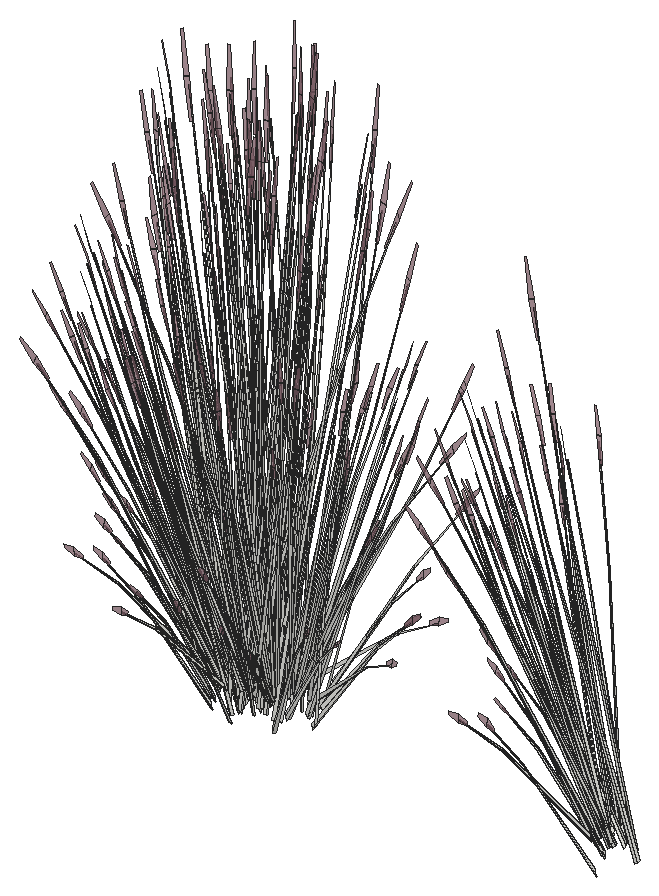
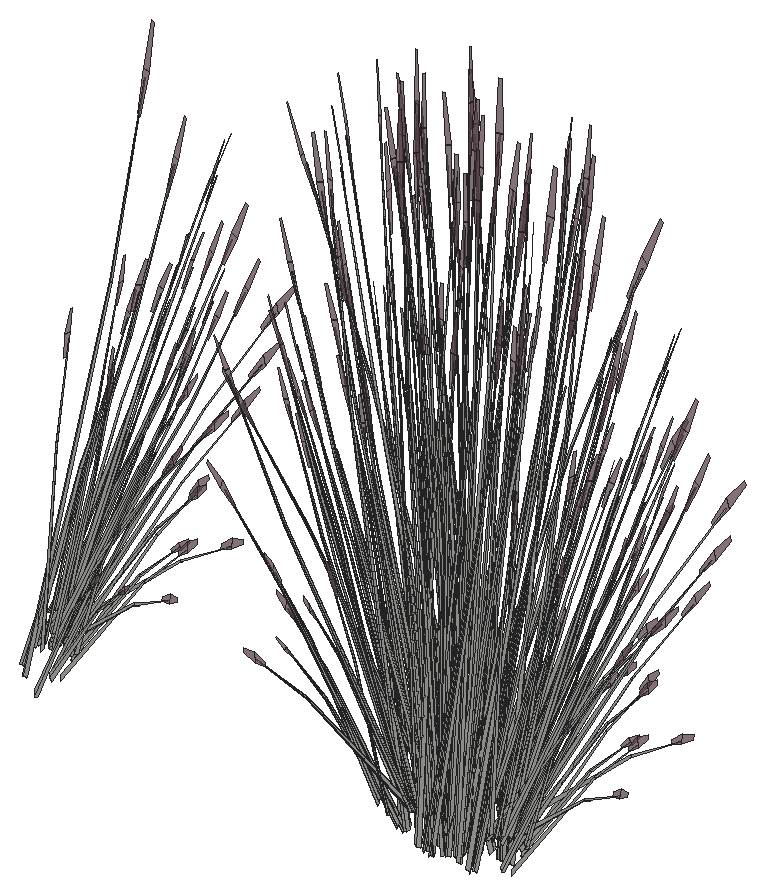
# SketchUp Ruby script. Lengths in inches.
U = 1.inch
M = Sketchup.active_model
def pt(a) = Geom::Point3d.new(a.map { |v| v * U })
def face(e, loops, mat)
  f = e.add_face(loops[0].map { |a| pt(a) })
  loops[1..].each { |l| e.add_face(l.map { |a| pt(a) }).erase! }
  f.material = f.back_material = mat if mat
  f
end
# faces: each face lists its corners as indices into pts; further lists are holes
def faces(e, pts, list, mat = nil) = list.each { |f| face(e, (f[0].is_a?(Array) ? f : [f]).map { |l| l.map { |i| pts[i] } }, mat) }
# xy, xz, yz: faces in a plane at the given z, y or x. An outline is a flat list of corners, or four numbers for a rectangle; further outlines are holes
def ring(l) = l.size == 4 ? [[l[0], l[1]], [l[2], l[1]], [l[2], l[3]], [l[0], l[3]]] : l.each_slice(2).to_a
def flat(e, list, mat, &to3) = list.each { |f| face(e, (f[0].is_a?(Array) ? f : [f]).map { |l| ring(l).map { |u, v| to3.(u, v) } }, mat) }
def xy(e, z, list, mat = nil) = flat(e, list, mat) { |x, y| [x, y, z] }
def xz(e, y, list, mat = nil) = flat(e, list, mat) { |x, z| [x, y, z] }
def yz(e, x, list, mat = nil) = flat(e, list, mat) { |y, z| [x, y, z] }
def lines(e, pts, list) = list.each { |a, b| e.add_line(pt(pts[a]), pt(pts[b])) }
# prism: a flat outline (further loops are holes) pulled along v
def prism(e, loops, v, mat = nil)
  f = face(e, loops, mat); d = Geom::Vector3d.new(v.map { |x| x * U })
  f.pushpull(f.normal.samedirection?(d) ? d.length : -d.length)
end
def box(e, o, s, mat = nil) = prism(e, [[o, [o[0] + s[0], o[1], o[2]], [o[0] + s[0], o[1] + s[1], o[2]], [o[0], o[1] + s[1], o[2]]]], [0, 0, s[2]], mat)
def at(x, y, z, deg = 0) = Geom::Transformation.translation(pt([x, y, z])) * Geom::Transformation.rotation(ORIGIN, Z_AXIS, deg.degrees)
def axes(o, x, y, z) = Geom::Transformation.new([*x, 0, *y, 0, *z, 0, *pt(o).to_a, 1])
def part(name) = M.definitions.add(name)
# library, detail: a bought-in or finely detailed component or shape, given as its bounding box
def library(name, o, s) = part(name).tap { |d| box(d.entities, o, s) }
def detail(e, o, s) = box(e.add_group.entities, o, s)
def put(e, d, t, mat = nil) = e.add_instance(d, t).tap { |i| i.material = mat if mat }
def group(e, t, mat = nil) = e.add_group.tap { |g| g.transformation = t; g.material = mat if mat }.entities
root = M.entities
M.materials.add("LightPink_Translucent").color = [144, 107, 117]
M.materials["LightPink_Translucent"].alpha = 0.75
c1 = part("blade")
p = [[2.15,0.21,22],[0,0.17,0],[0.09,0.45,0],[2.18,0.31,22],[2.29,0.31,22],[0.38,0.45,0],
  [2.48,0.24,33],[2.49,0.24,33],[2.48,0.22,33]]
faces(c1.entities,p,[[0,1,2,3],[4,5,2,3],[6,3,4,7],[8,0,3,6]])
c2 = part("seeds")
p = [[0.3,-0.1,1.38],[-0.01,-0.03,1.59],[-0.01,-0.03,0.03],[0.14,-0.07,-0.07],[0.29,-0.03,3],[0.15,0.01,3.11]]
faces(c2.entities,p,[[0,1,2,3],[1,0,4,5]],"LightPink_Translucent")
c3 = part("blade with seeds")
put(c3.entities,c1,at(0,0,0))
put(c3.entities,c2,axes([2.4,0.25,30.99],[1.5799,-0.05474,1.17369],[-0.12525,1.92788,0.29478],[-0.07173,-0.02425,1.56792]))
put(root,c3,axes([776.41,275.93,1.9375],[0.19062,-0.00741,0.85688],[-0.12645,0.32094,0.06928],[-0.27165,-0.01985,0.36631]))
put(root,c3,axes([776.49,276.49,1.9375],[0.15946,-0.06916,0.85688],[0.13424,0.31957,0.06928],[-0.25033,0.07223,0.36631]))
put(root,c3,axes([776,277.04,1.3],[0.15971,0.02684,0.71501],[0.10294,0.27415,-0.15377],[-0.21694,0.05132,0.3057]))
put(root,c3,axes([777.41,276.16,1.67],[0.13063,-0.0473,0.88532],[0.04505,0.33024,0.06928],[-0.28294,0.04382,0.31642]))
put(root,c3,axes([776,276.38,2.36],[-0.07505,0.04245,0.87472],[0.00638,0.31015,-0.13834],[-0.17202,0.04033,0.07015]))
put(root,c3,axes([776.98,275.63,2.49],[-0.45939,-0.00787,-0.35523],[0.03085,-0.3315,0.04287],[-0.19462,-0.03498,0.5025]))
put(root,c3,axes([776.61,275.71,1.3],[0.08973,0.09103,0.71501],[-0.20675,0.24743,-0.15377],[-0.2123,-0.05914,0.3057]))
put(root,c3,axes([776.25,276.21,2.26],[-0.38192,-0.09121,-0.17707],[0.11139,-0.2661,0.2286],[-0.15377,0.0244,0.4374]))
put(root,c3,axes([776.77,275.42,1.9375],[0.1707,0.05633,0.85688],[-0.35326,0.23632,0.06928],[-0.22018,-0.10661,0.36631]))
put(root,c3,axes([775.17,276.7,2.35],[0.05865,0.00877,0.88692],[0.18143,0.28888,-0.08381],[-0.12006,0.07582,0.15695]))
put(root,c3,axes([776.51,276.34,2.34],[-0.1245,0.29741,-0.25549],[-0.42685,-0.10194,-0.1979],[-0.17186,0.02727,0.48886]))
put(root,c3,axes([776.83,275.7,2.34],[-0.3337,0.21658,-0.25549],[-0.29224,-0.22879,-0.1979],[-0.16955,-0.03295,0.48886]))
put(root,c3,axes([776.29,276.32,0.75],[0.01165,0.05153,0.88171],[-0.23495,0.26909,-0.1347],[-0.16689,-0.01356,0.15018]))
put(root,c3,axes([776.36,275.09,2.35],[0.03407,0.03263,0.88692],[-0.16424,0.29331,-0.08381],[-0.16634,0.00212,0.15695]))
put(root,c3,axes([776.74,274.9,2.36],[-0.09888,-0.00231,0.87472],[-0.3148,0.23079,-0.13834],[-0.16797,-0.04716,0.07015]))
put(root,c3,axes([776.33,276.17,2.37],[0.12984,-0.29812,0.24001],[0.42685,0.10194,0.1979],[-0.16786,0.01792,0.49665]))
put(root,c3,axes([776.49,276.09,2.52],[0.23123,0.29606,-0.0608],[-0.41039,0.14549,-0.33747],[-0.17294,0.03906,0.51278]))
put(root,c3,axes([777.01,275.47,2.52],[-0.02461,0.33251,-0.0608],[-0.4659,-0.00909,-0.33747],[-0.17944,-0.0231,0.51278]))
put(root,c3,axes([776.71,275.5,2.26],[-0.26148,-0.20471,-0.17707],[0.29857,-0.19378,0.2286],[-0.1517,-0.02948,0.4374]))
put(root,c3,axes([776.3,276.09,2.37],[-0.16879,-0.22293,0.03215],[0.30779,-0.10912,0.2531],[-0.13568,0.02153,0.38595]))
put(root,c3,axes([776.08,275.99,1.38],[0.2934,-0.0234,0.5743],[-0.18611,0.20614,0.42196],[-0.14499,-0.03092,0.12649]))
put(root,c3,axes([776.4375,276.92,2.37],[-0.11397,-0.30091,0.24001],[0.44709,-0.05222,0.1979],[-0.13177,0.07077,0.49665]))
put(root,c3,axes([776.67,275.42,2.55],[0.37952,-0.24129,0.26881],[0.32731,0.25625,0.22165],[-0.17806,-0.04451,0.55625]))
put(root,c3,axes([776.35,276.86,2.37],[-0.31549,-0.13751,0.03215],[0.18368,-0.19581,0.2531],[-0.10115,0.06331,0.38595]))
put(root,c3,axes([776.65,276.18,2.53],[0.38192,0.09121,0.17707],[-0.11139,0.2661,-0.2286],[-0.15377,0.0244,0.4374]))
put(root,c3,axes([776.84,275.42,2.37],[0.02314,-0.24862,0.03215],[0.34943,0.00682,0.2531],[-0.13385,-0.02602,0.38595]))
put(root,c3,axes([777.83,276.79,1.03],[-0.47805,-0.0536,-0.31177],[0.10088,-0.33065,-0.08182],[-0.14266,-0.04007,0.68817]))
put(root,c3,axes([777.92,274.99,2.72],[-0.30671,0.31344,-0.0681],[-0.44417,-0.18058,-0.37797],[-0.1544,-0.08856,0.57432]))
put(root,c3,axes([777.08,275.6,2.53],[0.26148,0.20471,0.17707],[-0.29857,0.19378,-0.2286],[-0.1517,-0.02948,0.4374]))
put(root,c3,axes([777.78,275.24,2.49],[-0.39186,-0.15803,-0.35523],[0.27849,-0.27693,0.04287],[-0.14198,-0.09436,0.5025]))
put(root,c3,axes([777.6,275.25,2.34],[-0.45348,0.07772,-0.25549],[-0.07933,-0.29434,-0.1979],[-0.1218,-0.08435,0.48886]))
put(root,c3,axes([777.2,277.42,1.01],[-0.4301,-0.16348,-0.24825],[0.25708,-0.29314,0],[-0.09796,-0.03723,0.78752]))
put(root,c3,axes([777.01,274.98,0.75],[-0.04451,0.04307,0.88171],[-0.44986,0.09286,-0.1347],[-0.10868,-0.08448,0.15018]))
put(root,c3,axes([777.46,277.61,1.1875],[-0.28732,0.32763,0],[-0.4807,-0.18271,-0.25804],[-0.10948,-0.04161,0.81856]))
put(root,c3,axes([776.71,276.82,2.53],[0.40003,-0.04673,0.17707],[0.10563,0.26712,-0.2286],[-0.11464,0.07175,0.4374]))
put(root,c3,axes([776.73,275.15,1.0625],[-0.13257,0.26698,-0.01946],[-0.40802,-0.08212,-0.08825],[-0.06195,-0.04367,0.29107]))
put(root,c3,axes([777.8,274.24,2.35],[-0.00857,0.03919,0.88692],[-0.42284,0.14223,-0.08381],[-0.12443,-0.0727,0.15695]))
put(root,c3,axes([777.34,274.81,1.3],[-0.02783,0.10696,0.71501],[-0.40683,0.08954,-0.15377],[-0.0951,-0.13825,0.3057]))
put(root,c3,axes([777.48,275.09,1.9375],[0.10505,0.10498,0.85688],[-0.48542,0.08838,0.06928],[-0.10971,-0.1648,0.36631]))
put(root,c3,axes([778.37,276.84,1.33],[-0.46399,0.21707,-0.14548],[-0.30855,-0.30672,-0.25001],[-0.11448,-0.03115,0.79854]))
put(root,c3,axes([777.65,275.03,2.26],[-0.07098,-0.26335,-0.17707],[0.40574,-0.06954,0.2286],[-0.10898,-0.07547,0.4374]))
put(root,c3,axes([776.51,276.37,1.1875],[-0.57465,0,0],[0,-0.36542,-0.25804],[0,-0.08323,0.81856]))
put(root,c3,axes([777.32,277.29,1.01],[-0.10795,-0.28489,-0.15489],[0.42874,-0.0809,0.15489],[-0.08643,-0.03285,0.69487]))
put(root,c3,axes([777.89,275.25,2.53],[0.07098,0.26335,0.17707],[-0.40574,0.06954,-0.2286],[-0.10898,-0.07547,0.4374]))
put(root,c3,axes([776.96,276.27,1.17],[-0.42746,0.27488,0.15378],[-0.42772,-0.27199,-0.18246],[-0.01493,-0.07806,0.82443]))
put(root,c3,axes([778.72,277.03,1.66],[0.39713,0.13184,0.7563],[-0.38905,0.28403,0.29908],[-0.17427,-0.16834,0.63403]))
put(root,c3,axes([777.2,274.64,1.38],[0.23972,0.1138,0.5743],[-0.34912,0.06841,0.42196],[-0.0747,-0.08746,0.12649]))
put(root,c3,axes([778.89,276.9375,1.23],[-0.44875,-0.26316,-0.12596],[0.3776,-0.2955,0.27565],[-0.12084,0.03078,0.84108]))
put(root,c3,axes([778.08,276.68,1.11],[-0.27607,-0.27443,-0.2237],[0.41817,-0.19325,0.10766],[-0.08934,-0.03396,0.71822]))
put(root,c3,axes([777.7,274.9375,2.55],[0.51193,-0.08404,0.26881],[0.08885,0.32966,0.22165],[-0.1204,-0.09716,0.55625]))
put(root,c3,axes([778.67,276.88,1.11],[-0.49904,0.02018,-0.2237],[-0.04513,-0.33504,0.10766],[-0.08934,0.03396,0.71822]))
put(root,c3,axes([777.82,275.01,2.37],[0.20887,-0.2077,0.03215],[0.29744,0.12092,0.2531],[-0.09616,-0.06659,0.38595]))
put(root,c3,axes([777.71,277.44,1.24],[0.4301,0.16348,0.24825],[-0.25708,0.29314,0],[-0.09796,-0.03723,0.78752]))
put(root,c3,axes([778.12,276.84,1.22],[0.1218,-0.38743,-0.11714],[0.57753,0.06753,0.25635],[-0.10091,-0.0535,0.7822]))
put(root,c3,axes([778.33,276.93,1.31],[-0.08866,0.29179,0.0724],[-0.43315,-0.05065,-0.20674],[-0.07883,-0.02996,0.63372]))
put(root,c3,axes([778.28,274.39,2.36],[-0.07029,-0.04584,0.87472],[-0.46908,0.02906,-0.13834],[-0.07486,-0.10965,0.07015]))
put(root,c3,axes([776.64,276.12,1.01],[0,-0.32696,-0.24825],[0.51416,0,0],[0,-0.07447,0.78752]))
put(root,c3,axes([776.86,276.42,1.24],[0,0.32696,0.24825],[-0.51416,0,0],[0,-0.07447,0.78752]))
put(root,c3,axes([779.22,277.66,1.1],[-0.28374,-0.32877,-0.02571],[0.4807,-0.18271,0.25804],[-0.11845,0.0313,0.81815]))
put(root,c3,axes([779.09,277.62,1.01],[-0.42874,-0.0809,-0.15489],[0.10795,-0.28489,0.15489],[-0.08643,0.03285,0.69487]))
put(root,c3,axes([777.99,276.5,1.33],[-0.51755,-0.15601,-0.14548],[0.2492,-0.32927,-0.25001],[-0.01626,-0.08084,0.79854]))
put(root,c3,axes([777.76,276.16,1.05],[-0.18873,-0.33528,-0.34918],[0.54365,-0.12075,-0.09164],[-0.02086,-0.11353,0.77075]))
put(root,c3,axes([778.99,275.1,2.52],[-0.44971,0.15222,-0.0608],[-0.221,-0.27017,-0.33747],[-0.05933,-0.11385,0.51278]))
put(root,c3,axes([778.61,275.11,2.34],[-0.45175,-0.08196,-0.25549],[0.15485,-0.28101,-0.1979],[-0.04142,-0.11314,0.48886]))
put(root,c3,axes([776.86,276.125,1.01],[0.32079,-0.20399,-0.15489],[0.32079,0.20399,0.15489],[0,-0.06571,0.69487]))
put(root,c3,axes([778.3125,274.81,1.0625],[-0.31757,0.18757,-0.01946],[-0.29098,-0.20543,-0.08825],[-0.02049,-0.05821,0.29107]))
put(root,c3,axes([778.18,276.66,1.18],[0.58084,0.06889,0.22877],[-0.11821,0.38906,0.08977],[-0.08488,-0.03757,0.79428]))
put(root,c3,axes([778.03,276.59,1.36],[-0.22297,0.29461,0.2237],[-0.4633,-0.14179,-0.10766],[0,-0.06791,0.71822]))
put(root,c3,axes([778.77,275.17,2.49],[-0.21934,-0.26585,-0.35523],[0.45151,-0.14816,0.04287],[-0.05129,-0.12845,0.5025]))
put(root,c3,axes([777.87,277.28,1.24],[0.49383,-0.08678,0.08821],[0.12194,0.32295,0.17543],[-0.04404,-0.04705,0.80203]))
put(root,c3,axes([778.51,277.33,1.1],[-0.4633,-0.14679,0],[0.22297,-0.30501,0],[0,0,0.81353]))
put(root,c3,axes([778.86,275.2,2.53],[-0.13855,0.25143,0.17707],[-0.4042,-0.07334,-0.2286],[-0.03706,-0.10123,0.4374]))
put(root,c3,axes([779.34,277.29,1.24],[0.13276,-0.32494,0.08821],[0.4858,0.09195,0.17543],[-0.08392,0.00158,0.80203]))
put(root,c3,axes([779.12,276.86,1.31],[0.33952,0.19644,0.0724],[-0.2832,0.22163,-0.20674],[-0.07883,0.02996,0.63372]))
put(root,c3,axes([779,276.62,1.15],[-0.42746,-0.28142,-0.03066],[0.42772,-0.28159,0],[-0.01493,-0.00983,0.87786]))
put(root,c3,axes([779.11,276.72,1.36],[0.49904,-0.02018,0.2237],[0.04513,0.33504,-0.10766],[-0.08934,0.03396,0.71822]))
put(root,c3,axes([778.39,274.58,0.75],[-0.07708,0.01178,0.88171],[-0.42627,-0.1326,-0.1347],[0.00715,-0.1106,0.15018]))
put(root,c3,axes([779.48,277.47,1.24],[0.4301,-0.16348,0.24825],[0.25708,0.29314,0],[-0.09796,0.03723,0.78752]))
put(root,c3,axes([778.8125,274.94,2.26],[0.13855,-0.25143,-0.17707],[0.4042,0.07334,0.2286],[-0.03706,-0.10123,0.4374]))
put(root,c3,axes([778.13,276.3,1.18],[0.1998,0.3656,0.22877],[-0.5709,0.12713,0.08977],[0.00698,-0.06718,0.79428]))
put(root,c3,axes([778.04,276.25,1.11],[0.22297,-0.29461,-0.2237],[0.4633,0.14179,0.10766],[0,-0.06791,0.71822]))
put(root,c3,axes([778.61,277.2,1.1],[-0.14994,-0.28188,0],[0.42817,-0.09871,0],[0,0,0.77185]))
put(root,c3,axes([778.98,274.98,2.37],[0.33863,-0.11112,0.03215],[0.16575,0.20263,0.2531],[-0.0327,-0.08932,0.38595]))
put(root,c3,axes([780.1,276.47,1.24],[-0.36107,-0.23816,0.08821],[0.36387,-0.231,0.17543],[-0.03988,0.04864,0.80203]))
put(root,c3,axes([778.85,276.33,1.1],[0,-0.37831,0],[0.57465,0,0],[0,0,0.89728]))
put(root,c3,axes([778.86,275,2.37],[0.45283,0.08548,0.24001],[-0.15485,0.28101,0.1979],[-0.02721,-0.11051,0.49665]))
put(root,c3,axes([778.32,276.4,1.22],[0.5178,0.15847,0.12032],[-0.2492,0.32927,0.25001],[0,-0.0759,0.80271]))
put(root,c3,axes([779.14,276.48,1.15],[0,0.37813,-0.02818],[-0.57465,0,0],[0,0.01188,0.89684]))
put(root,c3,axes([778.15,276.18,1.36],[-0.49904,0.02018,0.2237],[-0.04513,-0.33504,-0.10766],[0.08934,-0.03396,0.71822]))
put(root,c3,axes([777.92,275.6,1.24],[-0.13276,0.32494,0.08821],[-0.4858,-0.09195,0.17543],[0.08392,-0.00158,0.80203]))
put(root,c3,axes([778.87,277.21,1.15],[0.1998,0.37562,-0.03006],[-0.5709,0.13162,0],[0.00698,0.01312,0.86086]))
put(root,c3,axes([777.68,275.2,1.1875],[-0.28732,-0.32763,0],[0.4807,-0.18271,-0.25804],[0.10948,-0.04161,0.81856]))
put(root,c3,axes([779.39,275.62,1.24],[-0.49383,0.08678,0.08821],[-0.12194,-0.32295,0.17543],[0.04404,0.04705,0.80203]))
put(root,c3,axes([778.88,274.41,1.38],[0.05895,0.19066,0.5743],[-0.32704,-0.1056,0.42196],[0.03519,-0.09762,0.12649]))
put(root,c3,axes([778.58,276.09,1.18],[-0.38104,0.29672,0.22877],[-0.45269,-0.26192,0.08977],[0.09186,-0.02961,0.79428]))
put(root,c3,axes([779.23,276.56,1.11],[0.32079,0.21119,0],[-0.32079,0.21119,0],[0,0,0.84633]))
put(root,c3,axes([779.23,276.3125,1.36],[0.22297,-0.29461,0.2237],[0.4633,0.14179,-0.10766],[0,0.06791,0.71822]))
put(root,c3,axes([779.03,277.33,1.1],[0.4633,0.14679,0],[-0.22297,0.30501,0],[0,0,0.87477]))
put(root,c3,axes([779.08,276.24,1.19],[-0.58084,-0.06889,0.24599],[0.11821,-0.38906,0.09653],[0.08488,0.03757,0.85407]))
put(root,c3,axes([780.29,274.72,2.35],[-0.04667,0.02497,0.88692],[-0.45726,-0.08426,-0.08381],[-0.01655,-0.10898,0.15695]))
put(root,c3,axes([779.93,275.44,2.52],[-0.50507,-0.0162,-0.0608],[0.01381,-0.30672,-0.33747],[0.03508,-0.11813,0.51278]))
put(root,c3,axes([779.24,276.41,1.1],[0.51416,0,0],[0,0.33849,0],[0,0,0.89203]))
put(root,c3,axes([779.73,275.49,2.53],[-0.31095,0.17214,0.17707],[-0.29435,-0.19656,-0.2286],[0.04479,-0.09987,0.4374]))
put(root,c3,axes([778.75,276.04,1.36],[-0.27607,-0.27443,0.2237],[0.41817,-0.19325,-0.10766],[0.08934,0.03396,0.71822]))
put(root,c3,axes([778.25,276.11,1.33],[-0.05355,-0.37308,-0.14548],[0.55775,-0.02256,-0.25001],[0.09822,-0.04969,0.79854]))
put(root,c3,axes([779.42,276.38,1.31],[0.42817,-0.09535,0.0724],[0.14994,0.27228,-0.20674],[0,0.05992,0.63372]))
put(root,c3,axes([779.58,275.33,2.34],[-0.32898,-0.21969,-0.25549],[0.34753,-0.1924,-0.1979],[0.05006,-0.11162,0.48886]))
put(root,c3,axes([778.17,275.28,1.01],[0.42874,0.0809,-0.15489],[-0.10795,0.28489,0.15489],[0.08643,-0.03285,0.69487]))
put(root,c3,axes([779.37,274.9375,1.3],[-0.13063,0.06618,0.71501],[-0.39122,-0.11583,-0.15377],[0.07252,-0.14406,0.3057]))
put(root,c3,axes([780.4,276.48,1.24],[0,-0.32696,0.24825],[0.51416,0,0],[0,0.07447,0.78752]))
put(root,c3,axes([778.07,275.15,1.01],[0.4301,-0.16348,-0.24825],[0.25708,0.29314,0],[0.09796,-0.03723,0.78752]))
put(root,c3,axes([778.93,275.96,1.31],[0.08866,-0.29179,0.0724],[0.43315,0.05065,-0.20674],[0.07883,0.02996,0.63372]))
put(root,c3,axes([779.55,275.45,1.24],[-0.4301,-0.16348,0.24825],[0.25708,-0.29314,0],[0.09796,0.03723,0.78752]))
put(root,c3,axes([779.68,275.43,2.49],[0.01196,-0.30243,-0.35523],[0.50354,0.02031,0.04287],[0.05314,-0.12813,0.5025]))
put(root,c3,axes([779.17,277.16,1.09],[0.48247,-0.11094,-0.09599],[0.16954,0.31956,0.00004],[0.05326,-0.01226,0.86949]))
put(root,c3,axes([779.18,276.21,1.11],[0.27607,0.27443,-0.2237],[-0.41817,0.19325,0.10766],[0.08934,0.03396,0.71822]))
put(root,c3,axes([779.89,275.24,2.26],[0.31095,-0.17214,-0.17707],[0.29435,0.19656,0.2286],[0.04479,-0.09987,0.4374]))
put(root,c3,axes([780.01,275.33,2.37],[0.37765,0.01523,0.03215],[-0.01035,0.23004,0.2531],[0.03952,-0.08812,0.38595]))
put(root,c3,axes([780.39,274.95,2.36],[-0.00444,-0.06507,0.87472],[-0.37468,-0.18807,-0.13834],[0.05793,-0.114,0.07015]))
put(root,c3,axes([778.58,275.82,1.03],[0.30954,-0.24575,-0.31177],[0.38452,0.22284,-0.08182],[0.12404,-0.0613,0.68817]))
put(root,c3,axes([779.89,275.3125,2.37],[0.32725,0.22308,0.24001],[-0.34753,0.1924,0.1979],[0.06036,-0.10466,0.49665]))
put(root,c3,axes([779.94,275.6,1.01],[0.10795,0.28489,-0.15489],[-0.42874,0.0809,0.15489],[0.08643,0.03285,0.69487]))
put(root,c3,axes([780.75,276.53,1.1875],[0.57465,0,0],[0,0.36542,-0.25804],[0,0.08323,0.81856]))
put(root,c3,axes([778.89,276.06,1.33],[0.46399,-0.21707,-0.14548],[0.30855,0.30672,-0.25001],[0.11448,0.03115,0.79854]))
put(root,c3,axes([780.27,276.02,2.53],[-0.40003,0.04673,0.17707],[-0.10563,-0.26712,-0.2286],[0.11464,-0.07175,0.4374]))
put(root,c3,axes([779.12,275.27,1.9375],[-0.08557,0.11238,0.85688],[-0.35897,-0.23257,0.06928],[0.16194,-0.14495,0.36631]))
put(root,c3,axes([777.72,275.86,0.8],[-0.45234,0.1309,0.64464],[-0.14398,-0.37559,0.25048],[0.27777,0.00625,0.73321]))
put(root,c3,axes([780.48,276.04,2.52],[-0.4251,-0.18028,-0.0608],[0.24491,-0.26108,-0.33747],[0.1201,-0.09075,0.51278]))
put(root,c3,axes([779.8,275.28,1.1875],[0.28732,-0.32763,0],[0.4807,0.18271,-0.25804],[0.10948,0.04161,0.81856]))
put(root,c3,axes([780.28,275.14,0.75],[-0.06878,-0.02576,0.88171],[-0.17668,-0.28776,-0.1347],[0.11919,-0.07809,0.15018]))
put(root,c3,axes([779.9,277.23,2.53],[-0.26148,-0.20471,0.17707],[0.29857,-0.19378,-0.2286],[0.1517,0.02948,0.4374]))
put(root,c3,axes([780.06,275.48,1.01],[0.4301,0.16348,-0.24825],[-0.25708,0.29314,0],[0.09796,0.03723,0.78752]))
put(root,c3,axes([780.26,275.83,2.34],[-0.11806,-0.29854,-0.25549],[0.44709,-0.05222,-0.1979],[0.12812,-0.08019,0.48886]))
put(root,c3,axes([781.05,277.37,1.96],[-0.08796,-0.27485,-0.01746],[0.41573,-0.06319,-0.07916],[0.08682,0.01742,0.26109]))
put(root,c3,axes([780.33,276.66,2.53],[-0.38192,-0.09121,0.17707],[0.11139,-0.2661,-0.2286],[0.15377,-0.0244,0.4374]))
put(root,c3,axes([779.43,276.11,1.03],[0.47805,0.0536,-0.31177],[-0.10088,0.33065,-0.08182],[0.14266,0.04007,0.68817]))
put(root,c3,axes([781.47,276.3,1.13],[-0.28491,-0.20907,-0.03244],[0.31204,-0.19157,-0.14708],[0.08842,-0.01349,0.48512]))
put(root,c3,axes([780.8125,275.24,1.38],[-0.15307,0.16644,0.5743],[-0.13157,-0.22361,0.42196],[0.12643,-0.05603,0.12649]))
put(root,c3,axes([780.63,275.98,2.37],[0.31549,0.13751,0.03215],[-0.18368,0.19581,0.2531],[0.10115,-0.06331,0.38595]))
put(root,c3,axes([780.54,275.92,2.37],[0.11397,0.30091,0.24001],[-0.44709,0.05222,0.1979],[0.13177,-0.07077,0.49665]))
put(root,c3,axes([781.52,275.97,2.35],[-0.06002,-0.00248,0.88692],[-0.24926,-0.26607,-0.08381],[0.1001,-0.08748,0.15695]))
put(root,c3,axes([780.59,275.86,2.26],[0.40003,-0.04673,-0.17707],[0.10563,0.26712,0.2286],[0.11464,-0.07175,0.4374]))
put(root,c3,axes([780.28,275.95,2.49],[0.24005,-0.25798,-0.35523],[0.42065,0.18334,0.04287],[0.14333,-0.09347,0.5025]))
put(root,c3,axes([780.68,276.74,2.37],[0.16879,0.22293,0.03215],[-0.30779,0.10912,0.2531],[0.13568,-0.02153,0.38595]))
put(root,c3,axes([779.97,277.36,2.52],[0.02461,-0.33251,-0.0608],[0.4659,0.00909,-0.33747],[0.17944,0.0231,0.51278]))
put(root,c3,axes([780.49,276.75,2.52],[-0.23123,-0.29606,-0.0608],[0.41039,-0.14549,-0.33747],[0.17294,-0.03906,0.51278]))
put(root,c3,axes([780.65,276.66,2.37],[-0.12984,0.29812,0.24001],[-0.42685,-0.10194,0.1979],[0.16786,-0.01792,0.49665]))
put(root,c3,axes([780.38,277.16,2.36],[0.09858,-0.00553,0.87472],[0.2704,-0.25401,-0.13834],[0.17535,0.03353,0.07015]))
put(root,c3,axes([780.47,276.49,2.34],[0.1245,-0.29741,-0.25549],[0.42685,0.10194,-0.1979],[0.17186,-0.02727,0.48886]))
put(root,c3,axes([781.54,276.68,1.38],[-0.28394,0.05398,0.5743],[0.13365,-0.22308,0.42196],[0.15063,0.01526,0.12649]))
put(root,c3,axes([780.625,275.71,1.3],[-0.16417,-0.00968,0.71501],[-0.16819,-0.25979,-0.15377],[0.20169,-0.07349,0.3057]))
put(root,c3,axes([780.73,276.63,2.26],[0.38192,0.09121,-0.17707],[-0.11139,0.2661,0.2286],[0.15377,-0.0244,0.4374]))
put(root,c3,axes([780,277.2,2.49],[0.45939,0.00787,-0.35523],[-0.03085,0.3315,0.04287],[0.19462,0.03498,0.5025]))
put(root,c3,axes([780.93,276.58,0.99],[-0.29599,0.03924,0.70792],[-0.04711,-0.31232,0.04052],[0.20731,-0.04727,0.40283]))
put(root,c3,axes([781.25,276.375,0.75],[-0.02402,-0.04964,0.88171],[0.16658,-0.29036,-0.1347],[0.16804,-0.00418,0.15018]))
put(root,c3,axes([781.41,277.63,2.35],[-0.04155,-0.02862,0.88692],[0.0909,-0.30682,-0.08381],[0.16368,-0.0196,0.15695]))
put(root,c3,axes([779.69,276.3,1.9375],[-0.19062,0.00741,0.85688],[0.12645,-0.32094,0.06928],[0.27165,0.01985,0.36631]))
put(root,c3,axes([780.39,276.6,2.49],[0.40382,-0.1444,-0.35523],[0.22505,0.29724,0.04287],[0.19512,-0.03377,0.5025]))
put(root,c3,axes([781.75,276.28,2.36],[0.06377,-0.0498,0.87472],[-0.08162,-0.30549,-0.13834],[0.16001,-0.05792,0.07015]))
put(root,c3,axes([781.01,277.04,1.3],[-0.11068,-0.08041,0.71501],[0.144,-0.26601,-0.15377],[0.22393,0.03604,0.3057]))
put(root,c3,axes([797.93,274.86,1.9375],[0.19062,-0.00741,0.85688],[-0.12645,0.32094,0.06928],[-0.27165,-0.01985,0.36631]))
put(root,c3,axes([798.01,275.43,1.9375],[0.15946,-0.06916,0.85688],[0.13424,0.31957,0.06928],[-0.25033,0.07223,0.36631]))
put(root,c3,axes([797.52,275.97,1.3],[0.15971,0.02684,0.71501],[0.10294,0.27415,-0.15377],[-0.21694,0.05132,0.3057]))
put(root,c3,axes([798.93,275.09,1.67],[0.13063,-0.0473,0.88532],[0.04505,0.33024,0.06928],[-0.28294,0.04382,0.31642]))
put(root,c3,axes([797.53,275.31,2.36],[-0.07505,0.04245,0.87472],[0.00638,0.31015,-0.13834],[-0.17202,0.04033,0.07015]))
put(root,c3,axes([798.5,274.5625,2.49],[-0.45939,-0.00787,-0.35523],[0.03085,-0.3315,0.04287],[-0.19462,-0.03498,0.5025]))
put(root,c3,axes([798.13,274.64,1.3],[0.08973,0.09103,0.71501],[-0.20675,0.24743,-0.15377],[-0.2123,-0.05914,0.3057]))
put(root,c3,axes([797.77,275.14,2.26],[-0.38192,-0.09121,-0.17707],[0.11139,-0.2661,0.2286],[-0.15377,0.0244,0.4374]))
put(root,c3,axes([798.29,274.35,1.9375],[0.1707,0.05633,0.85688],[-0.35326,0.23632,0.06928],[-0.22018,-0.10661,0.36631]))
put(root,c3,axes([796.69,275.63,2.35],[0.05865,0.00877,0.88692],[0.18143,0.28888,-0.08381],[-0.12006,0.07582,0.15695]))
put(root,c3,axes([798.03,275.27,2.34],[-0.1245,0.29741,-0.25549],[-0.42685,-0.10194,-0.1979],[-0.17186,0.02727,0.48886]))
put(root,c3,axes([798.35,274.63,2.34],[-0.3337,0.21658,-0.25549],[-0.29224,-0.22879,-0.1979],[-0.16955,-0.03295,0.48886]))
put(root,c3,axes([797.8125,275.26,0.75],[0.01165,0.05153,0.88171],[-0.23495,0.26909,-0.1347],[-0.16689,-0.01356,0.15018]))
put(root,c3,axes([797.88,274.02,2.35],[0.03407,0.03263,0.88692],[-0.16424,0.29331,-0.08381],[-0.16634,0.00212,0.15695]))
put(root,c3,axes([797.18,276.55,1.38],[0.19152,-0.14818,0.5743],[0.07557,0.23459,0.42196],[-0.13841,0.042,0.12649]))
put(root,c3,axes([798.26,273.83,2.36],[-0.09888,-0.00231,0.87472],[-0.3148,0.23079,-0.13834],[-0.16797,-0.04716,0.07015]))
put(root,c3,axes([797.86,275.1,2.37],[0.12984,-0.29812,0.24001],[0.42685,0.10194,0.1979],[-0.16786,0.01792,0.49665]))
put(root,c3,axes([798.01,275.02,2.52],[0.23123,0.29606,-0.0608],[-0.41039,0.14549,-0.33747],[-0.17294,0.03906,0.51278]))
put(root,c3,axes([798.53,274.4,2.52],[-0.02461,0.33251,-0.0608],[-0.4659,-0.00909,-0.33747],[-0.17944,-0.0231,0.51278]))
put(root,c3,axes([798.23,274.43,2.26],[-0.26148,-0.20471,-0.17707],[0.29857,-0.19378,0.2286],[-0.1517,-0.02948,0.4374]))
put(root,c3,axes([797.82,275.03,2.37],[-0.16879,-0.22293,0.03215],[0.30779,-0.10912,0.2531],[-0.13568,0.02153,0.38595]))
put(root,c3,axes([798.6,275.64,1.9375],[0.11478,-0.10046,0.85688],[0.28982,0.27117,0.06928],[-0.19878,0.12349,0.36631]))
put(root,c3,axes([797.91,275.91,2.26],[-0.40003,0.04673,-0.17707],[-0.10563,-0.26712,0.2286],[-0.11464,0.07175,0.4374]))
put(root,c3,axes([797.6875,276.7,0.75],[0.06164,0.03267,0.88171],[0.10452,0.30266,-0.1347],[-0.13662,0.06454,0.15018]))
put(root,c3,axes([797.6,274.92,1.38],[0.2934,-0.0234,0.5743],[-0.18611,0.20614,0.42196],[-0.14499,-0.03092,0.12649]))
put(root,c3,axes([797.96,275.85,2.37],[-0.11397,-0.30091,0.24001],[0.44709,-0.05222,0.1979],[-0.13177,0.07077,0.49665]))
put(root,c3,axes([798.1875,274.35,2.55],[0.37952,-0.24129,0.26881],[0.32731,0.25625,0.22165],[-0.17806,-0.04451,0.55625]))
put(root,c3,axes([797.87,275.79,2.37],[-0.31549,-0.13751,0.03215],[0.18368,-0.19581,0.2531],[-0.10115,0.06331,0.38595]))
put(root,c3,axes([798.17,275.11,2.53],[0.38192,0.09121,0.17707],[-0.11139,0.2661,-0.2286],[-0.15377,0.0244,0.4374]))
put(root,c3,axes([798.24,275.9375,2.34],[0.11806,0.29854,-0.25549],[-0.44709,0.05222,-0.1979],[-0.12812,0.08019,0.48886]))
put(root,c3,axes([798.36,274.35,2.37],[0.02314,-0.24862,0.03215],[0.34943,0.00682,0.2531],[-0.13385,-0.02602,0.38595]))
put(root,c3,axes([799.35,275.72,1.03],[-0.47805,-0.0536,-0.31177],[0.10088,-0.33065,-0.08182],[-0.14266,-0.04007,0.68817]))
put(root,c3,axes([799.4375,273.92,2.72],[-0.30671,0.31344,-0.0681],[-0.44417,-0.18058,-0.37797],[-0.1544,-0.08856,0.57432]))
put(root,c3,axes([798.6,274.53,2.53],[0.26148,0.20471,0.17707],[-0.29857,0.19378,-0.2286],[-0.1517,-0.02948,0.4374]))
put(root,c3,axes([799.3,274.17,2.49],[-0.39186,-0.15803,-0.35523],[0.27849,-0.27693,0.04287],[-0.14198,-0.09436,0.5025]))
put(root,c3,axes([799.12,274.18,2.34],[-0.45348,0.07772,-0.25549],[-0.07933,-0.29434,-0.1979],[-0.1218,-0.08435,0.48886]))
put(root,c3,axes([798.72,276.35,1.01],[-0.4301,-0.16348,-0.24825],[0.25708,-0.29314,0],[-0.09796,-0.03723,0.78752]))
put(root,c3,axes([798.53,273.91,0.75],[-0.04451,0.04307,0.88171],[-0.44986,0.09286,-0.1347],[-0.10868,-0.08448,0.15018]))
